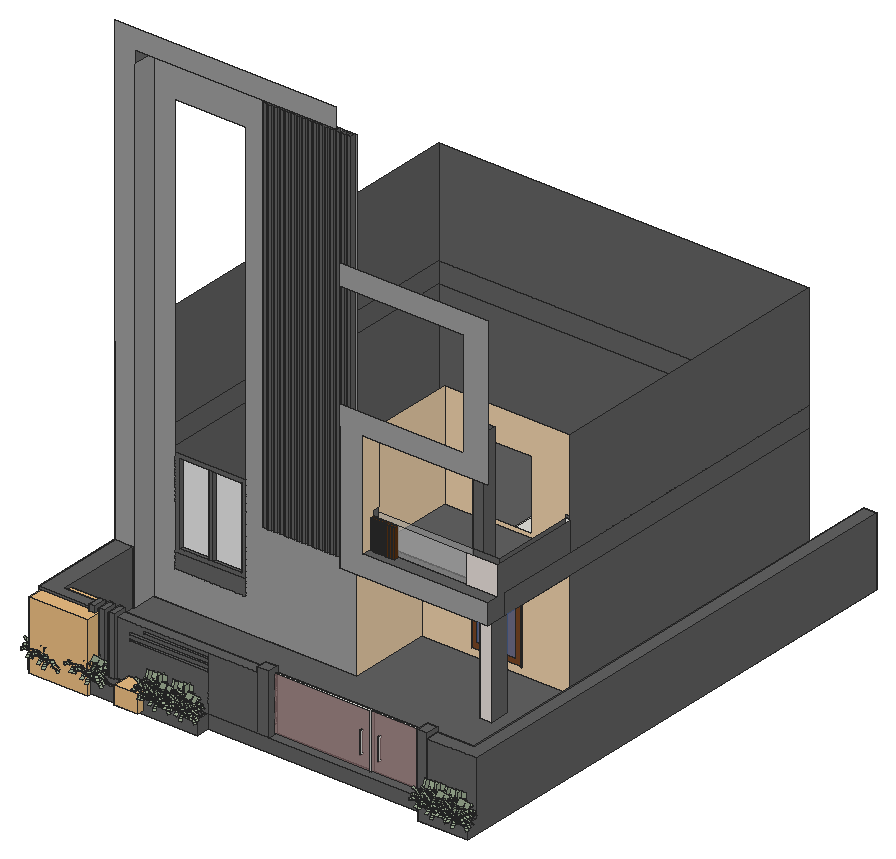
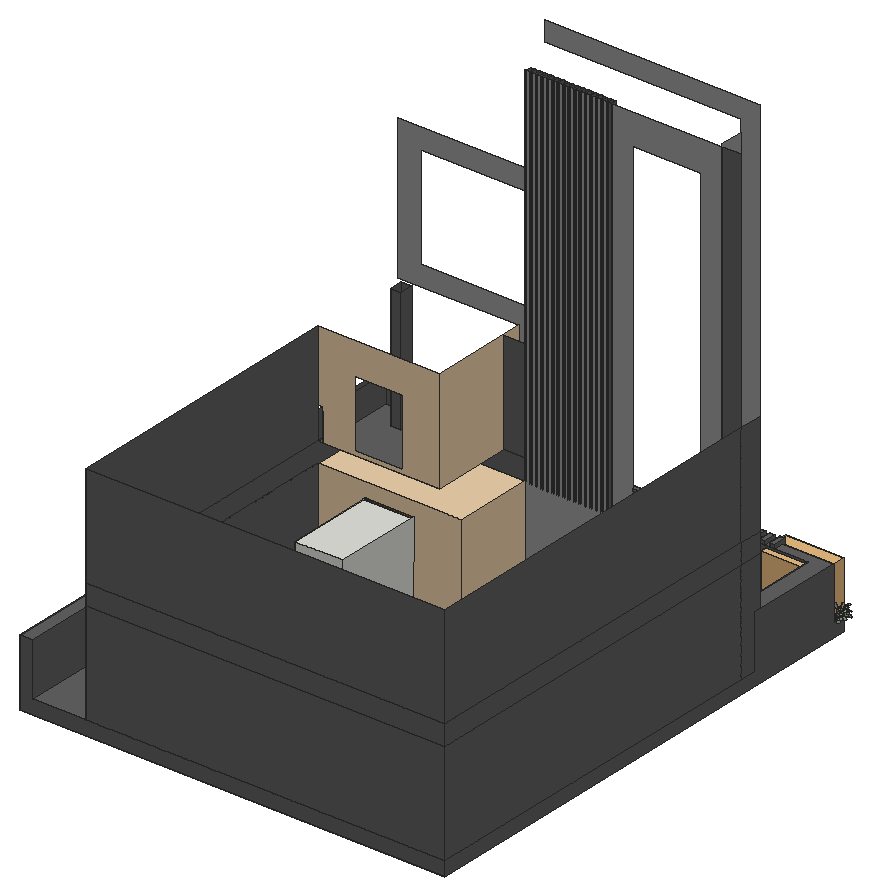
# SketchUp Ruby script. Lengths in inches.
U = 1.inch
M = Sketchup.active_model
def pt(a) = Geom::Point3d.new(a.map { |v| v * U })
def face(e, loops, mat)
  f = e.add_face(loops[0].map { |a| pt(a) })
  loops[1..].each { |l| e.add_face(l.map { |a| pt(a) }).erase! }
  f.material = f.back_material = mat if mat
  f
end
# faces: each face lists its corners as indices into pts; further lists are holes
def faces(e, pts, list, mat = nil) = list.each { |f| face(e, (f[0].is_a?(Array) ? f : [f]).map { |l| l.map { |i| pts[i] } }, mat) }
# xy, xz, yz: faces in a plane at the given z, y or x. An outline is a flat list of corners, or four numbers for a rectangle; further outlines are holes
def ring(l) = l.size == 4 ? [[l[0], l[1]], [l[2], l[1]], [l[2], l[3]], [l[0], l[3]]] : l.each_slice(2).to_a
def flat(e, list, mat, &to3) = list.each { |f| face(e, (f[0].is_a?(Array) ? f : [f]).map { |l| ring(l).map { |u, v| to3.(u, v) } }, mat) }
def xy(e, z, list, mat = nil) = flat(e, list, mat) { |x, y| [x, y, z] }
def xz(e, y, list, mat = nil) = flat(e, list, mat) { |x, z| [x, y, z] }
def yz(e, x, list, mat = nil) = flat(e, list, mat) { |y, z| [x, y, z] }
def lines(e, pts, list) = list.each { |a, b| e.add_line(pt(pts[a]), pt(pts[b])) }
# prism: a flat outline (further loops are holes) pulled along v
def prism(e, loops, v, mat = nil)
  f = face(e, loops, mat); d = Geom::Vector3d.new(v.map { |x| x * U })
  f.pushpull(f.normal.samedirection?(d) ? d.length : -d.length)
end
def box(e, o, s, mat = nil) = prism(e, [[o, [o[0] + s[0], o[1], o[2]], [o[0] + s[0], o[1] + s[1], o[2]], [o[0], o[1] + s[1], o[2]]]], [0, 0, s[2]], mat)
def at(x, y, z, deg = 0) = Geom::Transformation.translation(pt([x, y, z])) * Geom::Transformation.rotation(ORIGIN, Z_AXIS, deg.degrees)
def axes(o, x, y, z) = Geom::Transformation.new([*x, 0, *y, 0, *z, 0, *pt(o).to_a, 1])
def part(name) = M.definitions.add(name)
# library, detail: a bought-in or finely detailed component or shape, given as its bounding box
def library(name, o, s) = part(name).tap { |d| box(d.entities, o, s) }
def detail(e, o, s) = box(e.add_group.entities, o, s)
def put(e, d, t, mat = nil) = e.add_instance(d, t).tap { |i| i.material = mat if mat }
def group(e, t, mat = nil) = e.add_group.tap { |g| g.transformation = t; g.material = mat if mat }.entities
root = M.entities
M.materials.add("Generic\#1").color = [98, 98, 98]
M.materials.add("Generic\#2").color = [158, 158, 158]
M.materials.add("Generic\#3").color = [239, 209, 171]
M.materials.add("Generic\#4").color = [90, 50, 18]
M.materials.add("Generic\#5").color = [232, 223, 218]
M.materials.add("[Mirror 02]").color = [229, 229, 229]
M.materials.add("[Translucent Glass Blue]").color = [100, 149, 237]
M.materials["[Translucent Glass Blue]"].alpha = 0.5
M.materials.add("[Translucent Glass Gray]").color = [201, 201, 201]
M.materials["[Translucent Glass Gray]"].alpha = 0.5
M.materials.add("[Translucent Glass Gray]1").color = [142, 111, 111]
M.materials["[Translucent Glass Gray]1"].alpha = 0.81
M.materials.add("[Wood Veneer 01]").color = [120, 70, 37]
M.materials.add("hymenocallis littoralis").color = [156, 172, 146]
c1 = library("Flora+17",[-57.52,158.6,-38.64],[66.99,62.88,77.28])
c2 = library("Plante \#58",[-0.43,-1.58,0],[20.84,18.06,17.59])
c3 = part("Group\#856")
xy(c3.entities,7.38,[[0,0,5.5,15.91]],"hymenocallis littoralis")
p = [[5.5,28.78,0],[5.5,26.79,3.44],[0,26.79,3.44],[0,28.78,0],[0,23.75,6],[5.5,23.75,6],
  [0,15.91,7.38],[5.5,15.91,7.38]]
faces(c3.entities,p,[[0,1,2,3],[4,2,1,5],[6,4,5,7]],"hymenocallis littoralis")
c4 = part("Group\#854")
xy(c4.entities,7.38,[[0,0,5.5,15.91],[0,15.91,5.5,23.87]],"hymenocallis littoralis")
p = [[5.5,31.07,4.3],[5.5,27.74,6.47],[0,27.74,6.47],[0,31.07,4.3],[0,23.87,7.38],[5.5,23.87,7.38]]
faces(c4.entities,p,[[0,1,2,3],[4,2,1,5]],"hymenocallis littoralis")
c5 = part("Group\#857")
xy(c5.entities,7.38,[[0,0,5.6,15.91]],"hymenocallis littoralis")
p = [[5.6,28.78,0],[5.6,26.79,3.44],[0,26.79,3.44],[0,28.78,0],[0,23.75,6],[5.6,23.75,6],
  [0,15.91,7.38],[5.6,15.91,7.38]]
faces(c5.entities,p,[[0,1,2,3],[4,2,1,5],[6,4,5,7]],"hymenocallis littoralis")
c6 = part("Group\#855")
put(c6.entities,c4,axes([6.09,8.57,-0.52],[0.446,0.85617,0.26089],[-0.18444,-0.19731,0.96283],[0.87582,-0.47754,0.0699]))
put(c6.entities,c4,axes([6.29,7.28,-1.71],[0.37058,0.92707,-0.05667],[-0.32382,0.19004,0.99128],[0.87712,-0.32925,0.34964]))
put(c6.entities,c4,axes([11.04,16.14,-0.7],[1,0,0],[0,0.16628,1.02662],[0,-1.18456,0.19186]))
c7 = part("Group\#860")
put(c7.entities,c3,axes([24.57,32.05,-1.76],[0.9552,-0.22102,-0.19681],[0.4036,0.95545,0.88585],[-0.00568,-0.67859,0.7345]))
put(c7.entities,c3,axes([23.95,29.24,-2.4],[0,1,0],[-0.76041,0,0.64945],[0.64945,0,0.76041]))
put(c7.entities,c3,axes([24.22,24.72,-0.48],[-0.70711,0.70711,0],[-0.32757,-0.32757,0.80237],[0.61237,0.61237,0.5]))
put(c7.entities,c4,axes([20.66,37.22,-0.63],[1.12361,0.03262,0.39091],[-0.43499,0.29739,0.78777],[0.09852,-1.27434,0.37535]))
put(c7.entities,c3,axes([28.75,24.45,-2.4],[-1,0,0],[0,-0.76041,0.64945],[0,0.64945,0.76041]))
put(c7.entities,c5,axes([30.4,30.98,-3.7],[0.65676,-0.72002,0.22414],[0.55667,0.66341,0.5],[-0.50871,-0.20361,0.83652]))
put(c7.entities,c5,axes([32.41,29.61,-3.7],[0.04029,-0.97372,0.22414],[0.85287,0.15038,0.5],[-0.52057,0.17102,0.83652]))
put(c7.entities,c3,axes([31.89,25.85,-1.76],[-0.92056,0.33739,-0.19681],[-0.5186,-0.89824,0.88585],[0.08952,0.67268,0.7345]))
put(c7.entities,c3,axes([25.55,34.78,-0.48],[0.86603,0.5,0],[-0.25,0.43301,0.86603],[0.43301,-0.75,0.5]))
put(c7.entities,c5,axes([20.4,16.9375,-8.07],[-0.70711,0.70711,0],[-0.35754,-0.35754,0.65422],[1.3987,1.3987,1.52882]))
put(c7.entities,c3,axes([32.86,34.14,-0.48],[0.76604,-0.64279,0],[0.32139,0.38302,0.86603],[-0.55667,-0.66341,0.5]))
put(c7.entities,c3,axes([27.15,34.7,-0.1],[0.82472,-0.17528,-0.53769],[0.53769,0.53769,0.64945],[0.17528,-0.82472,0.53769]))
put(c7.entities,c3,axes([33.58,28.77,-2.4],[0,-1,0],[0.76041,0,0.64945],[-0.64945,0,0.76041]))
put(c7.entities,c3,axes([26.43,23.87,-2.81],[-0.75126,0.04415,0.65853],[0.53769,-0.53769,0.64945],[0.38276,0.84199,0.3802]))
put(c7.entities,c3,axes([28.78,23.98,-2.4],[-1,0,0],[0,-0.76041,0.64945],[0,0.64945,0.76041]))
put(c7.entities,c3,axes([25.39,25.38,-2.4],[-0.70711,0.70711,0],[-0.53769,-0.53769,0.64945],[0.45923,0.45923,0.76041]))
put(c7.entities,c3,axes([27.32,21.63,-0.1],[-0.45923,0.70711,-0.53769],[-0.76041,0,0.64945],[0.45923,0.70711,0.53769]))
put(c7.entities,c3,axes([25.17,27.625,-1.76],[0.56416,0.80187,-0.19681],[-0.66673,0.66673,0.80532],[0.62659,-0.26057,0.7345]))
put(c7.entities,c5,axes([27.59,27.04,-3.96],[-0.8993,-0.06127,0.43301],[0.2962,-0.8138,0.5],[0.32175,0.57791,0.75]))
put(c7.entities,c5,axes([26.98,24.5,-3.18],[-0.5,0.86603,0],[-0.75,-0.43301,0.5],[0.43301,0.25,0.86603]))
put(c7.entities,c5,axes([24.55,27.74,-3.7],[0.29517,0.92878,0.22414],[-0.85287,0.15038,0.5],[0.43068,-0.33875,0.83652]))
put(c7.entities,c5,axes([24.26,29.8,-3.18],[0.76604,0.64279,0],[-0.47317,0.5639,0.425],[0.32139,-0.38302,0.86603]))
put(c7.entities,c5,axes([25.98,32.46,-3.18],[1,0,0],[0,0.86603,0.5],[0,-0.5,0.86603]))
put(c7.entities,c3,axes([28.78,33.57,-2.4],[1,0,0],[0,0.76041,0.64945],[0,-0.64945,0.76041]))
put(c7.entities,c6,at(14.99,21.38,2.5))
put(c7.entities,c4,axes([34.63,26.34,-1.46],[-0.70089,-0.70877,0.07994],[0.4756,-0.38088,0.79293],[-0.53156,0.59378,0.60405]))
put(c7.entities,c4,axes([28.14,16.92,1.8125],[-1.19719,0.6912,0],[-0.09607,-0.16641,0.94244],[0.68444,1.18549,0.17613]))
put(c7.entities,c4,axes([31.5625,35.84,0.97],[0.66765,-1.1564,0.35779],[0.04445,0.30732,0.91033],[-1.20828,-0.64496,0.17012]))
put(c7.entities,c4,axes([38.94,22.51,0.89],[-0.97932,-0.67164,-0.05202],[0.27787,-0.41401,0.90999],[-0.85985,0.93577,0.32097]))
put(c7.entities,c4,axes([38.44,21.09,1.98],[-1.02864,-0.54856,0.2395],[0.33481,0.06999,0.88388],[-0.77261,1.08328,0.06417]))
put(c7.entities,c5,axes([35.02,30.51,-1.3],[-0.17365,-0.98481,0],[0.60224,-0.10619,0.79122],[-0.7792,0.13739,0.61153]))
put(c7.entities,c5,axes([29.41,22.33,-1.3],[-0.93969,0.34202,0],[-0.20915,-0.57465,0.79122],[0.27061,0.74351,0.61153]))
put(c7.entities,c4,axes([19.64,36,-1.62],[1.18194,0.09546,0.08234],[-0.14377,0.68823,0.76313],[0.21457,-1.1326,0.62386]))
put(c7.entities,c5,axes([24.25,24.14,-1.3],[-0.34202,0.93969,0],[-0.57465,-0.20915,0.79122],[0.74351,0.27061,0.61153]))
put(c7.entities,c5,axes([25.98,34.61,-1.3],[1,0,0],[0,0.61153,0.79122],[0,-0.79122,0.61153]))
put(c7.entities,c5,axes([31.16,34.41,-1.64],[0.56518,-0.80224,-0.19234],[0.73413,0.34233,0.72935],[-0.47639,-0.50772,0.71782]))
put(c7.entities,c5,axes([40.52,26.84,-5.82],[-0.42262,-0.90631,0],[0.48019,-0.22391,0.68552],[-1.43418,0.66877,1.22305]))
put(c7.entities,c3,axes([29.86,38.42,-1.01],[0.89064,-0.37013,0.26413],[-0.03924,0.63286,1.01918],[-0.45353,-0.76487,0.45748]))
put(c7.entities,c3,axes([29.34,22.4,-0.48],[-0.99619,-0.08716,0],[0.04358,-0.4981,0.86603],[-0.07548,0.86273,0.5]))
c8 = part("Group\#858")
xz(c8.entities,10.07,[[9.07,0,10.07,31.01],[0,31.01,0,45.12,20.13,45.12,20.13,31.01,10.07,31.01,10.07,32.58,9.07,32.58,9.07,31.01]],"hymenocallis littoralis")
yz(c8.entities,10.07,[[0,31.01,20.13,45.12]],"hymenocallis littoralis")
p = [[9.57,9.2,0],[10.07,10.07,0],[10.07,10.07,31.01],[10.07,10.07,32.58],[9.57,9.2,32.58]]
faces(c8.entities,p,[[0,1,2,3,4]],"hymenocallis littoralis")
c9 = part("cây lá nắng")
put(c9.entities,c7,axes([49.26,-2.75,0],[0.63109,0.63109,0],[-0.63109,0.63109,0],[0,0,0.935]))
g1 = group(c9.entities,at(26.6,-8.68,0))
put(g1,c3,axes([-4.72,35.73,-1.65],[0.74231,0.46334,-0.18402],[-0.34827,0.85768,0.82827],[0.42467,-0.43184,0.68675]))
put(g1,c3,axes([-3.34,33.57,-2.24],[-0.63109,0.63109,0],[-0.47989,-0.47989,0.60723],[0.40986,0.40986,0.71098]))
put(g1,c3,axes([-0.3125,30.89,-0.45],[-0.8925,0,0],[0,-0.41345,0.75022],[0,0.77293,0.4675]))
put(g1,c4,axes([-10.79,39.66,-0.59],[0.68852,0.72969,0.3655],[-0.4622,-0.08684,0.73657],[0.86641,-0.74205,0.35095]))
put(g1,c3,axes([2.71,33.57,-2.24],[-0.63109,-0.63109,0],[0.47989,-0.47989,0.60723],[-0.40986,0.40986,0.71098]))
put(g1,c5,axes([-0.37,38.74,-3.46],[0.86887,-0.03992,0.20957],[-0.06737,0.76999,0.4675],[-0.19255,-0.44954,0.78214]))
put(g1,c5,axes([1.76,39.14,-3.46],[0.63993,-0.58908,0.20957],[0.44333,0.63315,0.4675],[-0.43646,-0.2206,0.78214]))
put(g1,c3,axes([3.81,36.4375,-1.65],[-0.79389,-0.36803,-0.18402],[0.23959,-0.89415,0.82827],[-0.36803,0.48102,0.68675]))
put(g1,c3,axes([-5.83,38.07,-0.45],[0.231,0.86209,0],[-0.43104,0.1155,0.80973],[0.74659,-0.20005,0.4675]))
put(g1,c5,axes([2.18,23.5625,-7.55],[-0.8925,0,0],[0,-0.45128,0.6117],[0,1.76542,1.42944]))
put(g1,c3,axes([-0.8125,42.28,-0.45],[0.8891,0.07779,0],[-0.03889,0.44455,0.80973],[0.06737,-0.76999,0.4675]))
put(g1,c3,axes([-4.76,39.03,-0.09],[0.63109,0.40986,-0.50274],[0,0.67866,0.60723],[0.63109,-0.40986,0.50274]))
put(g1,c3,axes([3.03,39.35,-2.24],[0.63109,-0.63109,0],[0.47989,0.47989,0.60723],[-0.40986,-0.40986,0.71098]))
put(g1,c3,axes([1.61,31.74,-2.625],[-0.50198,-0.44625,0.61573],[0.67866,0,0.60723],[-0.28982,0.77293,0.35549]))
put(g1,c3,axes([3.03,33.3,-2.24],[-0.63109,-0.63109,0],[0.47989,-0.47989,0.60723],[-0.40986,0.40986,0.71098]))
put(g1,c3,axes([0.01,32.04,-2.24],[-0.8925,0,0],[0,-0.67866,0.60723],[0,0.57963,0.71098]))
put(g1,c3,axes([3.59,30.89,-0.09],[-0.73607,0.15643,-0.50274],[-0.47989,-0.47989,0.60723],[-0.15643,0.73607,0.50274]))
put(g1,c3,axes([-1.55,33.32,-1.65],[-0.15002,0.86209,-0.18402],[-0.84154,0,0.75297],[0.55988,0.231,0.68675]))
put(g1,c5,axes([0.35,34.48,-3.71],[-0.52887,-0.60621,0.40487],[0.70051,-0.32665,0.4675],[-0.16166,0.56777,0.70125]))
put(g1,c5,axes([2.61,39.13,-1.74],[-0.86209,0.231,0],[-0.23031,-0.85954,0.15531],[0.03162,0.11799,0.91645]))
put(g1,c5,axes([-2.02,33,-3.46],[-0.39986,0.77243,0.20957],[-0.63315,-0.44333,0.4675],[0.48558,0.05802,0.78214]))
put(g1,c5,axes([-3.49,34.12,-2.97],[0.07779,0.8891,0],[-0.65449,0.05726,0.39737],[0.44455,-0.03889,0.80973]))
put(g1,c5,axes([-4.09,36.88,-2.97],[0.63109,0.63109,0],[-0.54654,0.54654,0.4675],[0.31555,-0.31555,0.80973]))
put(g1,c3,axes([-3.02,39.35,-2.24],[0.63109,0.63109,0],[-0.47989,0.47989,0.60723],[0.40986,-0.40986,0.71098]))
put(g1,c6,axes([-4.03,22.95,2.33],[0.63109,0.63109,0],[-0.63109,0.63109,0],[0,0,0.935]))
put(g1,c4,axes([5.24,38.48,-1.37],[0.00497,-0.88963,0.07474],[0.54052,0.05978,0.74139],[-0.71019,0.03927,0.56479]))
put(g1,c4,axes([7.08,28.4375,1.7],[-1.19175,-0.31933,0],[0.04439,-0.16565,0.88118],[-0.31621,1.1801,0.16468]))
put(g1,c4,axes([-2.7,42.54,0.91],[1.15114,-0.30845,0.33454],[-0.1659,0.22199,0.85115],[-0.3555,-1.16957,0.15907]))
put(g1,c4,axes([10.37,38.78,0.83],[-0.19417,-1.04191,-0.04864],[0.43664,-0.08592,0.85084],[-1.1332,0.04791,0.30011]))
put(g1,c4,axes([10.95,37.5625,1.85],[-0.30298,-0.99536,0.22393],[0.16713,0.25547,0.82643],[-1.17124,0.19607,0.06]))
put(g1,c5,axes([2.84,41.36,-1.22],[0.51192,-0.73109,0],[0.44708,0.31305,0.73979],[-0.57846,-0.40504,0.57178]))
put(g1,c5,axes([4.47,32.65,-1.22],[-0.80888,-0.37719,0],[0.23066,-0.49465,0.73979],[-0.29844,0.64,0.57178]))
put(g1,c4,axes([-10.32,35.12,-1.51],[0.68567,0.80616,0.07699],[-0.52507,0.3436,0.71352],[0.85019,-0.57936,0.58331]))
put(g1,c5,axes([0.07,30.54,-1.22],[-0.80888,0.37719,0],[-0.23066,-0.49465,0.73979],[0.29844,0.64,0.57178]))
put(g1,c5,axes([-5.45,38.24,-1.22],[0.63109,0.63109,0],[-0.38593,0.38593,0.73979],[0.49934,-0.49934,0.57178]))
put(g1,c5,axes([-2.05,41.38,-1.53],[0.86296,-0.14961,-0.17984],[0.24726,0.67935,0.68194],[0.01977,-0.62107,0.67116]))
put(g1,c5,axes([8.63,42.51,-5.4375],[0.30525,-0.83868,0],[0.44435,0.16173,0.64096],[-1.32716,-0.48305,1.14356]))
put(g1,c3,axes([-5.4,43.09,-0.94],[0.79566,0.32849,0.24696],[-0.42416,0.37462,0.95293],[0.19648,-0.76892,0.42774]))
put(g1,c3,axes([4.38,32.65,-0.45],[-0.57369,-0.68369,0],[0.34185,-0.28684,0.80973],[-0.5921,0.49683,0.4675]))
put(g1,c5,axes([-2,33.84,-0.15],[-0.24601,0.85793,0],[-0.85539,-0.24528,0.15531],[0.11742,0.03367,0.91645]))
put(g1,c5,axes([0.17,30.83,-4.47],[-0.24601,0.85793,0],[-0.85539,-0.24528,0.15531],[0.11742,0.03367,0.91645]))
put(g1,c5,axes([-1.97,32.18,-4.47],[0.58524,0.67383,0],[-0.67184,0.58351,0.15531],[0.09222,-0.0801,0.91645]))
put(g1,c5,axes([-2,34.71,-4.47],[0.88392,-0.12346,0],[0.12309,0.88131,0.15531],[-0.0169,-0.12098,0.91645]))
put(g1,c5,axes([0.11,36.12,-4.47],[0.37822,-0.8084,0],[0.80601,0.37711,0.15531],[-0.11064,-0.05177,0.91645]))
put(c9.entities,c8,axes([29.71,14.29,6.94],[0.425,0.73612,0],[-0.6771,0.39092,-0.33349],[-0.26859,0.15507,0.72712]))
put(c9.entities,c8,axes([42.0625,26.12,6.94],[0.85,0,0],[0,0.78185,-0.33349],[0,0.33349,0.78185]))
put(c9.entities,c7,axes([7.3125,23.0625,0],[0.8925,0,0],[0,0.8925,0],[0,0,0.935]))
put(c9.entities,c8,axes([24.4375,40.23,2.05],[0.85,0,0],[0,0.85,0],[0,0,0.85]))
c10 = part("Planting+101")
put(c10.entities,c9,axes([21.34,32.96,-4.59],[0,-0.71,0],[-0.71,0,0],[0,0,0.71]))
c11 = part("Group\#1")
xy(c11.entities,0,[[0,0,1.25,2.55]])
xy(c11.entities,1.125,[[0,1.125,1.25,2.55]])
xy(c11.entities,23.91,[[0,1.125,1.25,2.55]])
xy(c11.entities,25.04,[[0,0,1.25,2.55]])
xz(c11.entities,0,[[0,0,1.25,25.04]])
xz(c11.entities,1.125,[[0,1.125,1.25,23.91]])
yz(c11.entities,0,[[0,0,0,25.04,2.55,25.04,2.55,23.91,1.125,23.91,1.125,1.125,2.55,1.125,2.55,0]])
yz(c11.entities,1.25,[[0,0,2.55,0,2.55,1.125,1.125,1.125,1.125,23.91,2.55,23.91,2.55,25.04,0,25.04]])
c12 = part("Group\#6")
xy(c12.entities,0,[[0,0,56.6875,3.1875]],"[Wood Veneer 01]")
xy(c12.entities,78.875,[[0,0,56.6875,3.1875]],"[Wood Veneer 01]")
xz(c12.entities,0,[[5.8,5.8,28.34,73.07],[31.82,5.8,50.88,73.07]],"[Translucent Glass Blue]")
xz(c12.entities,0,[[[0,0,56.6875,78.875],[5.8,5.8,50.88,73.07]],[28.34,5.8,31.82,73.07]],"[Wood Veneer 01]")
xz(c12.entities,3.1875,[[0,0,56.6875,78.875]],"[Wood Veneer 01]")
yz(c12.entities,0,[[0,0,3.1875,78.875]],"[Wood Veneer 01]")
yz(c12.entities,56.6875,[[0,0,3.1875,78.875]],"[Wood Veneer 01]")
c13 = part("Group\#4")
xy(c13.entities,32.5625,[[0,0,2.875,5]])
xz(c13.entities,0,[[0,0,2.875,32.5625]])
yz(c13.entities,0,[[0,0,5,32.5625]])
yz(c13.entities,2.875,[[0,0,5,32.5625]])
xy(root,-15.9375,[[9.73,12.88,9.73,595.51,506.85,595.51,506.85,15.2,450.85,15.2,450.85,27.82,201.83,27.82,201.83,12.88]],"Generic\#1")
xy(root,-13.25,[[11.85,15.01,199.7,25.7]],"Generic\#1")
xy(root,-11.5625,[[452.21,16.56,505.49,26.46]],"Generic\#1")
xy(root,0,[[9.73,12.88,201.83,12.88,201.83,27.82,98.44,27.82,98.44,25.7,199.7,25.7,199.7,15.01,11.85,15.01,11.85,25.7,69.36,25.7,69.36,27.82,9.73,27.82],[[11.85,15.01,199.7,25.7],[11.85,15.01,199.7,15.01,199.7,25.7,98.44,25.7,98.44,24.51,92.11,24.51,92.11,25.7,87.07,25.7,87.07,24.51,80.73,24.51,80.73,25.7,75.69,25.7,75.69,24.51,69.36,24.51,69.36,25.7,11.85,25.7]],[[450.85,15.2,506.85,27.82],[452.21,16.56,505.49,26.46]],[69.36,24.51,75.69,25.7],[80.73,24.51,87.07,25.7],
  [92.11,24.51,98.44,25.7],[69.36,25.7,75.69,27.82],[75.69,25.7,80.73,27.82],[80.73,25.7,87.07,27.82],[87.07,25.7,92.11,27.82],
  [92.11,25.7,98.44,27.82],[[271.48,27.82,439.48,27.82,439.48,42.63,492.35,42.63,492.35,595.51,429.73,595.51,429.73,256.07,262.1,256.07,262.1,163.51,32.23,163.51,32.23,136.13,30.16,136.13,30.16,39.51,271.48,39.51],[395.47,172.46,408.85,194.1]],[439.48,27.82,450.85,42.63],[30.16,136.13,32.23,136.13,32.23,163.51,9.73,163.51,9.73,143.07,30.16,143.07],[9.73,163.51,262.1,163.51,262.1,256.07,429.73,256.07,429.73,595.51,9.73,595.51]],"Generic\#1")
xy(root,7.5,[[318.61,256.07,374.42,359.51]])
xy(root,42.35,[[112.7,27.82,201.83,39.51]],"Generic\#1")
xy(root,44.96,[[112.7,27.82,201.83,39.51]],"Generic\#1")
xy(root,48.97,[[112.7,27.82,201.83,39.51]],"Generic\#1")
xy(root,51.58,[[112.7,27.82,201.83,39.51]],"Generic\#1")
xy(root,55.41,[[128.76,27.82,201.83,39.51]],"Generic\#1")
xy(root,58.02,[[128.76,27.82,201.83,39.51]],"Generic\#1")
xy(root,58.89,[[61.12,163.51,94.41,167.88],[98.41,163.51,131.71,167.88]],"Generic\#1")
xy(root,62.0625,[[9.73,27.82,69.36,27.82,69.36,39.51,30.16,39.51,30.16,136.13,9.73,136.13],[69.36,27.82,75.69,39.51],[75.69,27.82,80.73,39.51],[80.73,27.82,87.07,39.51],[87.07,27.82,92.11,39.51],
  [92.11,27.82,98.44,39.51],[98.44,27.82,257.73,39.51],[450.85,27.82,506.85,27.82,506.85,595.51,492.35,595.51,492.35,42.63,450.85,42.63],[9.73,136.13,30.16,143.07]],"Generic\#1")
xy(root,66.375,[[69.36,24.51,75.69,39.51],[80.73,24.51,87.07,39.51],[92.11,24.51,98.44,39.51]],"Generic\#1")
xy(root,67.25,[[257.73,27.82,271.48,39.51],[439.48,27.82,450.85,42.63]],"Generic\#1")
xy(root,103.22,[[318.3125,256.07,374.125,359.51]])
xy(root,118.23,[[160.6,157.13,164.98,163.51]],"Generic\#1")
xy(root,120,[[262.1,139.95,429.73,163.51],[262.1,163.51,429.73,256.07]],"Generic\#3")
xy(root,120.8125,[[395.47,172.46,408.85,194.1]],"Generic\#1")
xy(root,143.5,[[287.79,139.95,429.73,139.95,429.73,153.95,292.35,153.95,292.35,148.95,289.48,148.95,289.48,153.95,287.79,153.95],[289.48,148.95,292.35,153.95],[[287.79,163.51,424.66,256.07],[383.97,176.93,396.09,192.68]],[424.66,163.51,429.73,256.07],[383.97,176.93,396.09,192.68]],"Generic\#1")
xz(root,12.88,[[9.73,-15.9375,201.83,0]],"Generic\#1")
xz(root,15.01,[[11.85,-13.25,199.7,0]],"Generic\#1")
xz(root,15.2,[[450.85,-15.9375,506.85,0]],"Generic\#1")
xz(root,16.56,[[452.21,-11.5625,505.49,0]],"Generic\#1")
xz(root,24.51,[[69.36,0,75.69,66.375],[80.73,0,87.07,66.375],[92.11,0,98.44,66.375]],"Generic\#1")
xz(root,25.7,[[11.85,-13.25,199.7,0]],"Generic\#1")
xz(root,26.46,[[452.21,-11.5625,505.49,0]],"Generic\#1")
xz(root,27.82,[[201.83,-15.9375,450.85,0],[9.73,0,69.36,62.0625],[69.36,0,75.69,62.0625],[75.69,0,80.73,62.0625],[80.73,0,87.07,62.0625],
  [87.07,0,92.11,62.0625],[92.11,0,98.44,62.0625],[98.44,0,201.83,0,201.83,42.35,112.7,42.35,112.7,44.96,201.83,44.96,201.83,48.97,112.7,48.97,112.7,51.58,201.83,51.58,201.83,55.41,128.76,55.41,128.76,58.02,201.83,58.02,201.83,62.0625,98.44,62.0625],[201.83,0,257.73,62.0625],[257.73,0,271.48,67.25],
  [439.48,0,450.85,67.25],[450.85,0,506.85,62.0625]],"Generic\#1")
xz(root,39.51,[[[30.16,0,30.16,62.0625,257.73,62.0625,257.73,67.25,271.48,67.25,271.48,0],[112.7,48.97,201.83,51.58],[112.7,42.35,201.83,44.96],[128.76,55.41,201.83,58.02]],[69.36,62.0625,75.69,66.375],[80.73,62.0625,87.07,66.375],[92.11,62.0625,98.44,66.375]],"Generic\#1")
xz(root,42.63,[[439.48,0,450.85,67.25],[450.85,0,492.35,62.0625]],"Generic\#1")
xz(root,136.13,[[30.16,0,32.23,0,32.23,568.125,260.65,568.125,260.65,590.5625,9.73,590.5625,9.73,62.0625,30.16,62.0625]],"Generic\#2")
xz(root,139.95,[[262.1,120,429.73,120,429.73,143.5,287.79,143.5,287.79,263.5,429.73,263.5,429.73,430.5,262.1,430.5,262.1,407,403.16,407,403.16,287,262.1,287]],"Generic\#2")
xz(root,143.07,[[9.73,0,30.16,62.0625]],"Generic\#1")
xz(root,153.95,[[287.79,143.5,289.48,176.0625],[289.48,143.5,292.35,176.0625]],"Generic\#1")
xz(root,153.95,[[395.15,143.5,429.73,176.0625]],"Generic\#5")
xz(root,153.95,[[292.35,143.5,395.15,176.0625]],"[Translucent Glass Gray]")
xz(root,157.13,[[160.6,118.23,164.98,550.5],[166.98,118.23,171.35,550.5],[173.35,118.23,177.73,550.5],[179.73,118.23,184.1,550.5],[186.1,118.23,190.48,550.5],
  [192.48,118.23,196.85,550.5],[198.85,118.23,203.23,550.5],[205.23,118.23,209.6,550.5],[211.6,118.23,215.98,550.5],[217.98,118.23,222.35,550.5],
  [224.35,118.23,228.73,550.5],[230.73,118.23,235.1,550.5],[237.1,118.23,241.48,550.5],[243.48,118.23,247.85,550.5],[249.85,118.8,254.23,550.5],
  [256.23,118.9,260.6,550.5]],"Generic\#1")
xz(root,163.51,[[9.73,0,32.23,550.5],[160.6,0,164.98,0.01],[56.23,36,136.6,54],[[56.23,54,136.6,155.625],[61.12,58.89,131.71,150.73]],[94.41,58.89,98.41,150.73],
  [160.6,118.23,164.98,550.5],[262.1,120,429.73,143.5],[262.1,143.5,287.79,263.5],[395.15,143.5,424.66,176.0625]],"Generic\#1")
xz(root,163.51,[[[32.23,0,160.6,0,160.6,0.01,164.98,0.01,164.98,0,262.1,0,262.1,550.5,164.98,550.5,164.98,118.23,160.6,118.23,160.6,550.5,32.23,550.5],[56.23,36,136.6,514.5]]],"Generic\#2")
xz(root,163.51,[[287.79,143.5,395.15,176.0625]],"[Translucent Glass Gray]")
xz(root,167.88,[[61.12,58.89,94.41,150.73],[98.41,58.89,131.71,150.73]],"[Mirror 02]")
xz(root,172.46,[[395.47,0,408.85,120.8125]],"Generic\#5")
xz(root,176.93,[[383.97,143.5,396.09,287]],"Generic\#1")
xz(root,192.68,[[383.97,143.5,396.09,287]],"Generic\#1")
xz(root,194.1,[[395.47,0,408.85,120.8125]],"Generic\#1")
xz(root,256.07,[[[262.1,0,429.73,120],[318.61,7.5,318.3125,103.22,374.125,103.22,374.42,7.5]],[[287.79,143.5,424.66,143.5,424.66,180.875,429.73,180.875,429.73,263.5,287.79,263.5],[330.78,147.94,387.47,226.82]]],"Generic\#3")
xz(root,359.51,[[318.61,7.5,374.42,7.5,374.125,103.22,318.3125,103.22]])
xz(root,595.51,[[9.73,-15.9375,9.73,0,492.35,0,492.35,62.0625,506.85,62.0625,506.85,-15.9375],[9.73,0,429.73,120],[9.73,120,429.73,143.5],[9.73,143.5,429.73,263.5]],"Generic\#1")
yz(root,9.73,[[12.88,-15.9375,12.88,0,27.82,0,27.82,62.0625,143.07,62.0625,143.07,0,595.51,0,595.51,-15.9375],[143.07,0,143.07,62.0625,136.13,62.0625,136.13,120,163.51,120,163.51,0],[163.51,0,595.51,120],[136.13,120,163.51,143.5],[163.51,120,595.51,143.5],
  [136.13,143.5,163.51,263.5],[163.51,143.5,595.51,263.5]],"Generic\#1")
yz(root,11.85,[[15.01,-13.25,25.7,0]],"Generic\#1")
yz(root,30.16,[[39.51,0,136.13,62.0625],[136.13,0,143.07,62.0625]],"Generic\#1")
yz(root,32.23,[[136.13,0,163.51,553.3125]],"Generic\#2")
yz(root,61.12,[[163.51,58.89,167.88,150.73]],"Generic\#1")
yz(root,69.36,[[24.51,0,24.51,66.375,39.51,66.375,39.51,62.0625,27.82,62.0625,27.82,0]],"Generic\#1")
yz(root,75.69,[[24.51,0,27.82,0,27.82,62.0625,39.51,62.0625,39.51,66.375,24.51,66.375]],"Generic\#1")
yz(root,80.73,[[24.51,0,24.51,66.375,39.51,66.375,39.51,62.0625,27.82,62.0625,27.82,0]],"Generic\#1")
yz(root,87.07,[[24.51,0,27.82,0,27.82,62.0625,39.51,62.0625,39.51,66.375,24.51,66.375]],"Generic\#1")
yz(root,92.11,[[24.51,0,24.51,66.375,39.51,66.375,39.51,62.0625,27.82,62.0625,27.82,0]],"Generic\#1")
yz(root,94.41,[[163.51,58.89,167.88,150.73]],"Generic\#1")
yz(root,98.41,[[163.51,58.89,167.88,150.73]],"Generic\#1")
yz(root,98.44,[[24.51,0,27.82,0,27.82,62.0625,39.51,62.0625,39.51,66.375,24.51,66.375]],"Generic\#1")
yz(root,112.7,[[27.82,42.35,39.51,44.96],[27.82,48.97,39.51,51.58]],"Generic\#1")
yz(root,128.76,[[27.82,55.41,39.51,58.02]],"Generic\#1")
yz(root,131.71,[[163.51,58.89,167.88,150.73]],"Generic\#1")
yz(root,160.6,[[157.13,118.23,163.51,550.5]],"Generic\#1")
yz(root,164.98,[[157.13,118.23,163.51,550.5]],"Generic\#1")
yz(root,166.98,[[157.13,118.23,163.51,550.5]],"Generic\#1")
yz(root,171.35,[[157.13,118.23,163.51,550.5]],"Generic\#1")
yz(root,173.35,[[157.13,118.23,163.51,550.5]],"Generic\#1")
yz(root,177.73,[[157.13,118.23,163.51,550.5]],"Generic\#1")
yz(root,179.73,[[157.13,118.23,163.51,550.5]],"Generic\#1")
yz(root,184.1,[[157.13,118.23,163.51,550.5]],"Generic\#1")
yz(root,186.1,[[157.13,118.23,163.51,550.5]],"Generic\#1")
yz(root,190.48,[[157.13,118.23,163.51,550.5]],"Generic\#1")
yz(root,192.48,[[157.13,118.23,163.51,550.5]],"Generic\#1")
yz(root,196.85,[[157.13,118.23,163.51,550.5]],"Generic\#1")
yz(root,198.85,[[157.13,118.23,163.51,550.5]],"Generic\#1")
yz(root,199.7,[[15.01,-13.25,25.7,0]],"Generic\#1")
yz(root,201.83,[[12.88,-15.9375,27.82,0],[27.82,42.35,39.51,44.96],[27.82,48.97,39.51,51.58],[27.82,55.41,39.51,58.02]],"Generic\#1")
yz(root,203.23,[[157.13,118.23,163.51,550.5]],"Generic\#1")
yz(root,205.23,[[157.13,118.23,163.51,550.5]],"Generic\#1")
yz(root,209.6,[[157.13,118.23,163.51,550.5]],"Generic\#1")
yz(root,211.6,[[157.13,118.23,163.51,550.5]],"Generic\#1")
yz(root,215.98,[[157.13,118.23,163.51,550.5]],"Generic\#1")
yz(root,217.98,[[157.13,118.23,163.51,550.5]],"Generic\#1")
yz(root,222.35,[[157.13,118.23,163.51,550.5]],"Generic\#1")
yz(root,224.35,[[157.13,118.23,163.51,550.5]],"Generic\#1")
yz(root,228.73,[[157.13,118.23,163.51,550.5]],"Generic\#1")
yz(root,230.73,[[157.13,118.23,163.51,550.5]],"Generic\#1")
yz(root,235.1,[[157.13,118.23,163.51,550.5]],"Generic\#1")
yz(root,237.1,[[157.13,118.23,163.51,550.5]],"Generic\#1")
yz(root,241.48,[[157.13,118.23,163.51,550.5]],"Generic\#1")
yz(root,243.48,[[157.13,118.23,163.51,550.5]],"Generic\#1")
yz(root,247.85,[[157.13,118.23,163.51,550.5]],"Generic\#1")
yz(root,249.85,[[157.13,118.8,163.51,550.5]],"Generic\#1")
yz(root,254.23,[[157.13,118.8,163.51,550.5]],"Generic\#1")
yz(root,256.23,[[157.13,118.9,163.51,550.5]],"Generic\#1")
yz(root,257.73,[[27.82,62.0625,39.51,67.25]],"Generic\#1")
yz(root,260.6,[[157.13,118.9,163.51,550.5]],"Generic\#1")
yz(root,262.1,[[139.95,120,163.51,143.5],[139.95,143.5,163.51,263.5]],"Generic\#1")
yz(root,262.1,[[163.51,0,256.07,120]],"Generic\#3")
yz(root,271.48,[[27.82,0,39.51,67.25]],"Generic\#1")
yz(root,287.79,[[139.95,143.5,153.95,143.5,153.95,180.875,163.51,180.875,163.51,263.5,139.95,263.5],[163.51,143.5,256.07,263.5]],"Generic\#3")
yz(root,383.97,[[176.93,143.5,192.68,287]],"Generic\#1")
yz(root,395.47,[[172.46,0,194.1,120.8125]],"Generic\#1")
yz(root,396.09,[[176.93,143.5,192.68,287]],"Generic\#1")
yz(root,408.85,[[172.46,0,194.1,120.8125]],"Generic\#1")
yz(root,424.66,[[163.51,143.5,256.07,176.0625]],"Generic\#1")
yz(root,429.73,[[256.07,0,595.51,120],[139.95,120,163.51,120,163.51,143.5,256.07,143.5,256.07,176.0625,153.95,176.0625,153.95,143.5,139.95,143.5],[163.51,120,595.51,143.5],[256.07,143.5,595.51,263.5]],"Generic\#1")
yz(root,439.48,[[27.82,0,42.63,67.25]],"Generic\#1")
yz(root,450.85,[[15.2,-15.9375,27.82,0],[27.82,0,42.63,62.0625],[27.82,62.0625,42.63,67.25]],"Generic\#1")
yz(root,452.21,[[16.56,-11.5625,26.46,0]],"Generic\#1")
yz(root,492.35,[[42.63,0,595.51,62.0625]],"Generic\#1")
yz(root,505.49,[[16.56,-11.5625,26.46,0]],"Generic\#1")
yz(root,506.85,[[15.2,-15.9375,595.51,-15.9375,595.51,62.0625,27.82,62.0625,27.82,0,15.2,0]],"Generic\#1")
p = [[318.3125,256.07,103.22],[318.61,256.07,7.5],[318.61,359.51,7.5],[318.3125,359.51,103.22],[374.42,256.07,7.5],[374.125,256.07,103.22],
  [374.125,359.51,103.22],[374.42,359.51,7.5]]
faces(root,p,[[0,1,2,3],[4,5,6,7]])
put(root,c1,axes([70.09,-85.12,21.09],[1,0,0],[0,0.6,0],[0,0,1]))
put(root,c2,axes([113.47,7.75,-12.58],[1.2996,0,0],[0,1.14,0],[0,0,1.14]))
put(root,c10,axes([17.15,15.68,-0.7],[0,-0.7347,0],[0.93,0,0],[0,0,0.93]))
put(root,c10,axes([143.08,15.68,1.3],[0,-0.7347,0],[0.93,0,0],[0,0,0.93]))
put(root,c10,axes([172.65,15.68,1.3],[0,-0.7347,0],[0.93,0,0],[0,0,0.93]))
put(root,c10,axes([458.02,15.68,1.3],[0,-0.7347,0],[0.93,0,0],[0,0,0.93]))
put(root,c10,axes([481.9,15.68,1.3],[0,-0.7347,0],[0.93,0,0],[0,0,0.93]))
put(root,c10,axes([66.33,15.68,1.3],[0,-0.7347,0],[0.93,0,0],[0,0,0.93]))
g2 = group(root,at(271.48,32.68,0))
xy(g2,0,[[0,2.55,108.3125,5.68],[110.3125,2.55,168,5.68]])
xy(g2,62.0625,[[0,2.55,108.3125,5.68],[110.3125,2.55,168,5.68]])
xz(g2,2.55,[[99.2,39.04,100.45,40.17]])
xz(g2,2.55,[[[0,0,108.3125,62.0625],[99.2,39.04,100.45,40.17],[99.2,15.125,100.45,16.25]],[110.3125,0,168,62.0625]],"[Translucent Glass Gray]1")
xz(g2,5.68,[[0,0,108.3125,62.0625],[108.3125,0,110.3125,62.0625],[110.3125,0,168,62.0625]])
yz(g2,0,[[2.55,0,5.68,62.0625]])
yz(g2,108.3125,[[2.55,0,5.68,62.0625]])
yz(g2,110.3125,[[2.55,0,5.68,62.0625]])
yz(g2,168,[[2.55,0,5.68,62.0625]])
p = [[99.76,0.55,15.68],[99.76,2.55,15.68],[99.76,0.55,39.61],[99.76,2.55,39.61]]
lines(g2,p,[[0,1],[2,0],[3,2]])
put(g2,c11,at(119.08,0,15.125))
put(g2,c11,at(99.2,0,15.125))
put(root,c12,axes([318.61,256.07,7.5],[1,0,0],[0,1,0],[0,0,1.21357]))
put(root,c13,at(289.48,148.95,143.5),"Generic\#4")
put(root,c13,at(292.98,148.95,143.5),"Generic\#4")
put(root,c13,at(296.48,148.95,143.5),"Generic\#4")
put(root,c13,at(299.98,148.95,143.5),"Generic\#4")
put(root,c13,at(303.48,148.95,143.5),"Generic\#4")
put(root,c13,at(306.98,148.95,143.5),"Generic\#4")
put(root,c13,at(310.48,148.95,143.5),"Generic\#4")
put(root,c13,at(313.98,148.95,143.5),"Generic\#4")
